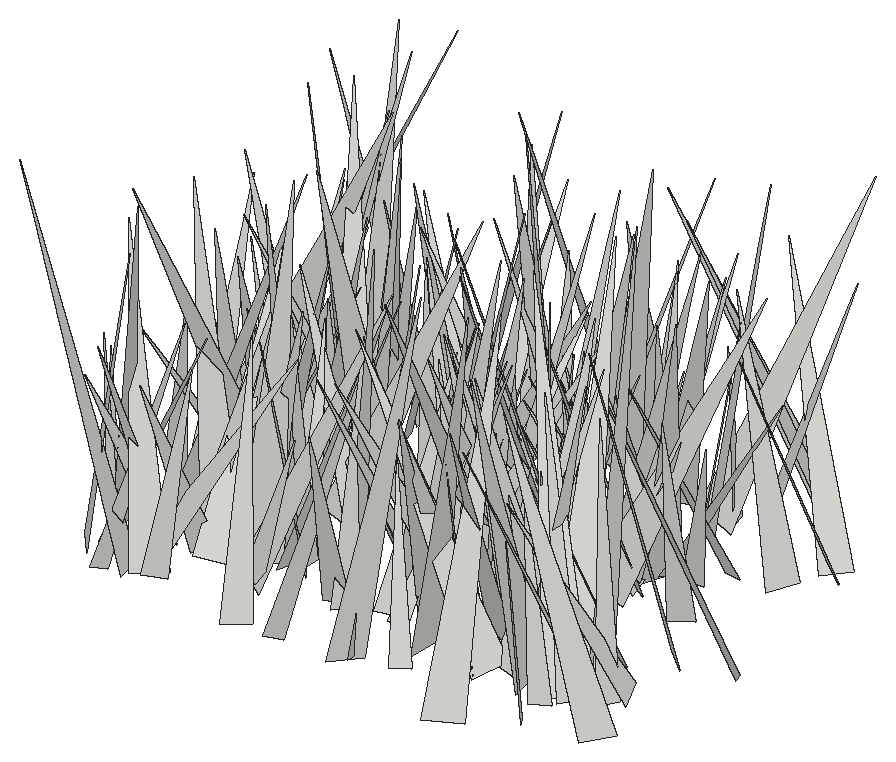
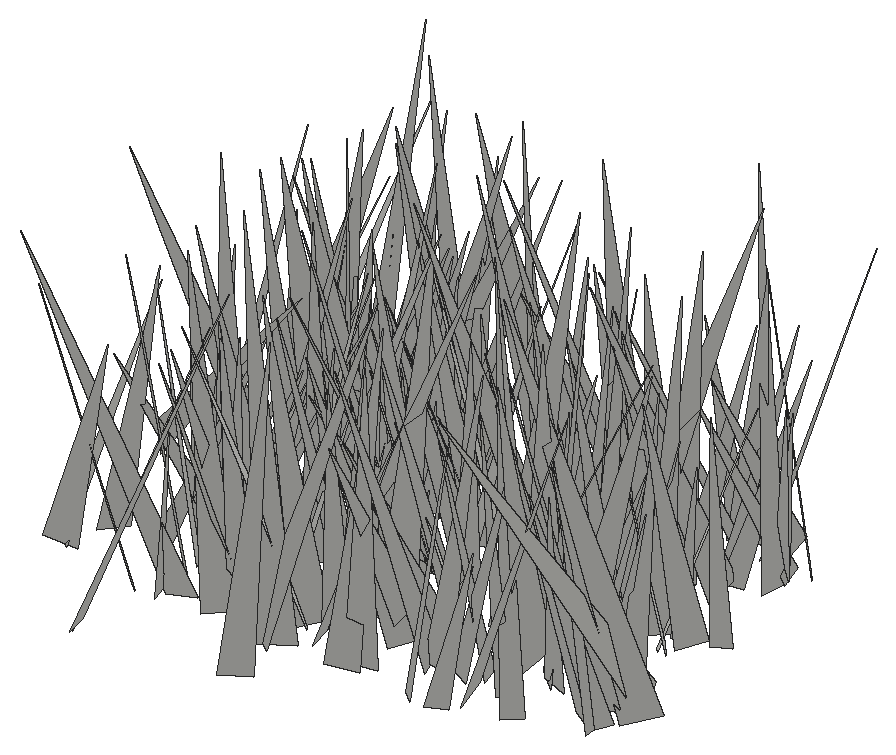
# SketchUp Ruby script. Lengths in inches.
U = 1.inch
M = Sketchup.active_model
def pt(a) = Geom::Point3d.new(a.map { |v| v * U })
def face(e, loops, mat)
  f = e.add_face(loops[0].map { |a| pt(a) })
  loops[1..].each { |l| e.add_face(l.map { |a| pt(a) }).erase! }
  f.material = f.back_material = mat if mat
  f
end
# faces: each face lists its corners as indices into pts; further lists are holes
def faces(e, pts, list, mat = nil) = list.each { |f| face(e, (f[0].is_a?(Array) ? f : [f]).map { |l| l.map { |i| pts[i] } }, mat) }
# xy, xz, yz: faces in a plane at the given z, y or x. An outline is a flat list of corners, or four numbers for a rectangle; further outlines are holes
def ring(l) = l.size == 4 ? [[l[0], l[1]], [l[2], l[1]], [l[2], l[3]], [l[0], l[3]]] : l.each_slice(2).to_a
def flat(e, list, mat, &to3) = list.each { |f| face(e, (f[0].is_a?(Array) ? f : [f]).map { |l| ring(l).map { |u, v| to3.(u, v) } }, mat) }
def xy(e, z, list, mat = nil) = flat(e, list, mat) { |x, y| [x, y, z] }
def xz(e, y, list, mat = nil) = flat(e, list, mat) { |x, z| [x, y, z] }
def yz(e, x, list, mat = nil) = flat(e, list, mat) { |y, z| [x, y, z] }
def lines(e, pts, list) = list.each { |a, b| e.add_line(pt(pts[a]), pt(pts[b])) }
# prism: a flat outline (further loops are holes) pulled along v
def prism(e, loops, v, mat = nil)
  f = face(e, loops, mat); d = Geom::Vector3d.new(v.map { |x| x * U })
  f.pushpull(f.normal.samedirection?(d) ? d.length : -d.length)
end
def box(e, o, s, mat = nil) = prism(e, [[o, [o[0] + s[0], o[1], o[2]], [o[0] + s[0], o[1] + s[1], o[2]], [o[0], o[1] + s[1], o[2]]]], [0, 0, s[2]], mat)
def at(x, y, z, deg = 0) = Geom::Transformation.translation(pt([x, y, z])) * Geom::Transformation.rotation(ORIGIN, Z_AXIS, deg.degrees)
def axes(o, x, y, z) = Geom::Transformation.new([*x, 0, *y, 0, *z, 0, *pt(o).to_a, 1])
def part(name) = M.definitions.add(name)
# library, detail: a bought-in or finely detailed component or shape, given as its bounding box
def library(name, o, s) = part(name).tap { |d| box(d.entities, o, s) }
def detail(e, o, s) = box(e.add_group.entities, o, s)
def put(e, d, t, mat = nil) = e.add_instance(d, t).tap { |i| i.material = mat if mat }
def group(e, t, mat = nil) = e.add_group.tap { |g| g.transformation = t; g.material = mat if mat }.entities
root = M.entities
c1 = part("fur_instance\#9")
p = [[0.8125,0,1.79],[0.67,-0.02,1.48],[0,-0.11,0],[0,0.11,0]]
faces(c1.entities,p,[[0,1,2,3]])
put(root,c1,axes([133.73,308.41,-27.1],[-4.47092,-4.93614,0.16266],[-4.90041,4.46105,0.68268],[0.61475,-0.33851,6.62484]))
put(root,c1,axes([114.86,306.08,-27.1],[-2.17172,3.54056,2.13295],[3.72846,2.71807,-0.7156],[1.78427,-1.37037,4.09143]))
put(root,c1,axes([130.49,308.72,-27.1],[7.53052,-1.13144,2.64431],[-0.30654,-7.68469,-2.41514],[-2.85982,-2.15562,7.22191]))
put(root,c1,axes([113.78,305.95,-27.1],[-7.70081,-2.50661,0.76749],[-2.60656,7.57519,-1.4131],[0.27927,1.58364,7.97425]))
put(root,c1,axes([119.4,305.24,-27.1],[3.60121,-2.60608,3.3834],[-3.59297,-4.24118,0.55747],[-2.30861,2.53545,4.41017]))
put(root,c1,axes([132.16,306.06,-27.1],[-3.20539,-1.99252,1.2784],[-2.28309,3.17085,-0.78241],[0.62603,1.36182,3.69222]))
put(root,c1,axes([135.17,306.77,-27.1],[-3.75455,5.21199,1.89568],[5.51913,3.28609,1.89629],[-0.5456,-2.62523,6.13723]))
put(root,c1,axes([124.23,305.61,-27.1],[6.87844,-2.02965,2.77665],[-2.6588,-7.07628,1.41394],[-2.18175,2.22463,7.03088]))
put(root,c1,axes([111.28,306.52,-27.1],[4.60486,4.04407,1.88978],[4.30358,-4.74303,-0.33665],[-1.18533,-1.50984,6.1193]))
put(root,c1,axes([113.47,308.5,-27.1],[-0.2394,-4.99537,0.47277],[-5.01072,0.21306,-0.28607],[-0.26442,0.48521,4.99291]))
put(root,c1,axes([129.92,304.25,-27.1],[-5.97227,4.9002,0.90124],[4.6479,5.98621,-1.7477],[1.79477,0.80344,7.52499]))
put(root,c1,axes([111.55,308.375,-27.1],[7.9282,0.66664,2.15118],[1.11346,-8.00329,-1.62351],[-1.9576,-1.85234,7.78877]))
put(root,c1,axes([114.93,308.92,-27.1],[3.23703,-3.40023,0.62778],[-3.13183,-3.24768,-1.44163],[-1.46538,-0.57015,4.46784]))
put(root,c1,axes([112.91,309.12,-27.1],[3.29812,-3.00828,0.87507],[-2.53709,-3.30998,-1.81667],[-1.83812,-0.82908,4.07763]))
put(root,c1,axes([121.28,308.8,-27.1],[1.53045,-4.60076,0.23907],[-4.60681,-1.52625,0.11946],[0.03806,0.26453,4.84716]))
put(root,c1,axes([114.52,306.23,-27.1],[-3.46559,5.8146,1.30946],[5.95968,3.40104,0.67057],[0.08042,-1.46897,6.73574]))
put(root,c1,axes([126.2,306.37,-27.1],[-1.47936,3.73163,0.54523],[3.76451,1.42617,0.45319],[-0.22551,-0.67216,3.98851]))
put(root,c1,axes([128.33,307.89,-27.1],[-3.06281,-3.15709,1.43812],[-3.29391,3.24851,0.11628],[1.08883,0.94666,4.3971]))
put(root,c1,axes([127.84,310.375,-27.1],[-0.91329,-6.82842,0.06821],[-6.63421,0.90353,1.6239],[1.61843,-0.14959,6.69511]))
put(root,c1,axes([112.84,305.34,-27.1],[4.59265,0.40937,1.72839],[-0.43371,-4.3881,2.19176],[-1.72245,2.19644,4.05662]))
put(root,c1,axes([125.98,308.26,-27.1],[7.89082,-0.9052,1.78608],[-0.78265,-8.07818,-0.63641],[-1.84308,-0.44515,7.91703]))
put(root,c1,axes([113.76,307.28,-27.1],[3.2036,5.15972,0.63397],[4.7617,-2.61371,-2.78969],[2.08586,-1.95793,5.39475]))
put(root,c1,axes([131.92,307.42,-27.1],[-1.38179,3.78074,1.32931],[4.00762,1.30133,0.46468],[-0.00636,-1.40818,3.99842]))
put(root,c1,axes([112.24,306.98,-27.1],[0.5553,3.90242,1.15183],[3.90207,-0.84018,0.96535],[-1.15302,-0.96393,3.8217]))
put(root,c1,axes([117.9,308.01,-27.1],[1.20072,-3.47995,0.99765],[-3.52529,-0.88496,1.15597],[0.82322,1.28603,3.49507]))
put(root,c1,axes([111.97,307.41,-27.1],[0.50374,3.60666,1.32904],[3.78488,-0.69911,0.46265],[-0.67011,-1.23747,3.61216]))
put(root,c1,axes([128.89,308.32,-27.1],[-6.43604,2.78332,0.65453],[2.85741,6.20344,1.71766],[-0.1023,-1.83529,6.79846]))
put(root,c1,axes([124.49,310.56,-27.1],[6.011,-2.52803,0.45147],[-2.2406,-5.7244,-2.22212],[-1.25478,-1.8887,6.13068]))
put(root,c1,axes([134.04,310.125,-27.1],[-4.91943,-1.92287,0.32626],[-1.70701,4.67316,1.80343],[0.9434,-1.57124,4.96446]))
put(root,c1,axes([126.09,310.48,-27.1],[4.34994,-4.04005,0.73934],[-3.73736,-4.34022,-1.72779],[-1.70317,-0.79441,5.67968]))
put(root,c1,axes([121.12,305.25,-27.1],[5.49101,0.89671,2.25711],[-0.37206,-5.20349,2.97239],[-2.40004,2.85822,4.70322]))
put(root,c1,axes([124.3,306.1,-27.1],[-6.72177,-1.11045,3.37602],[-2.29516,6.87097,-2.30972],[2.71346,3.06096,6.4094]))
put(root,c1,axes([125.15,311.5,-27.1],[-6.3203,-1.31951,1.76492],[-0.3807,5.93404,3.07318],[2.17051,-2.80147,5.67828]))
put(root,c1,axes([111.65,307.2,-27.1],[4.45385,0.90104,0.34779],[0.77968,-4.32278,1.21461],[-0.57002,1.12752,4.37874]))
put(root,c1,axes([117.67,308.17,-27.1],[3.41975,6.53108,1.33927],[6.45057,-2.86091,-2.51965],[1.68487,-2.30293,6.92828]))
put(root,c1,axes([123.74,311.39,-27.1],[-5.24067,-3.21189,0.67738],[-2.84495,5.08085,2.08111],[1.63749,-1.45206,5.78359]))
put(root,c1,axes([121.59,309.46,-27.1],[-3.32783,-6.52848,3.29816],[-6.89122,4.01297,0.99019],[2.45153,2.41834,7.26051]))
put(root,c1,axes([118.82,310.05,-27.1],[-3.91635,-3.27614,1.36892],[-3.24396,4.13005,0.60351],[1.44353,0.39293,5.07017]))
put(root,c1,axes([121.82,308.65,-27.1],[4.3952,-2.19196,2.60814],[-2.70598,-4.83259,0.49862],[-2.06997,1.6632,4.88608]))
put(root,c1,axes([123.3,310.01,-27.1],[3.09975,-1.98369,0.33098],[-1.98147,-3.11644,-0.1208],[-0.34401,0.07615,3.67817]))
put(root,c1,axes([117.23,309.3,-27.1],[-5.12716,5.45276,3.67809],[5.84452,5.9162,-0.62364],[3.01704,-2.19425,7.45865]))
put(root,c1,axes([132.65,308.37,-27.1],[-5.52094,1.92393,0.48296],[1.85996,5.5174,-0.71721],[0.68943,0.52184,5.80241]))
put(root,c1,axes([129.99,309.48,-27.1],[5.84499,-0.86217,1.83487],[-1.09003,-6.05756,0.62599],[-1.70936,0.91471,5.87498]))
put(root,c1,axes([116.05,310.88,-27.1],[3.45559,-4.90486,0.92565],[-4.98413,-3.32981,0.96246],[0.2699,1.30779,5.9222]))
put(root,c1,axes([118.2,309.93,-27.1],[6.4862,-0.82849,0.61771],[-0.87391,-6.49276,0.46816],[-0.55158,0.54452,6.52212]))
put(root,c1,axes([124.09,308.82,-27.1],[-0.30009,3.62925,0.24074],[3.53668,0.34756,-0.831],[0.84929,-0.16496,3.54556]))
put(root,c1,axes([115.39,312.97,-27.1],[0.76231,-8.24421,0.75454],[-8.09051,-0.90251,-1.68715],[-1.75496,0.57958,8.10565]))
put(root,c1,axes([133.84,309.01,-27.1],[-5.20641,1.3754,0.94823],[1.21962,5.25029,-0.91901],[1.14166,0.66356,5.30602]))
put(root,c1,axes([132.34,308.51,-27.1],[-4.81407,6.51041,0.79127],[6.55623,4.75265,0.78417],[-0.16528,-1.10168,8.05889]))
put(root,c1,axes([114.375,309.32,-27.1],[1.48764,5.46016,1.29529],[5.56167,-1.25605,-1.09283],[0.74757,-1.52092,5.55267]))
put(root,c1,axes([129.38,308.63,-27.1],[1.31333,6.20143,0.89],[6.24264,-1.21867,-0.72041],[0.52849,-1.01577,6.2979]))
put(root,c1,axes([114.73,310.27,-27.1],[-4.39266,5.33205,2.64396],[5.82364,4.52851,0.54275],[1.2274,-2.40386,6.88706]))
put(root,c1,axes([125.45,313.41,-27.1],[-0.22294,-7.81188,0.28991],[-7.80547,0.20653,-0.4373],[-0.42917,0.30182,7.80282]))
put(root,c1,axes([123.33,309.29,-27.1],[-3.03856,4.16793,1.35783],[3.96538,3.31773,-1.3102],[1.86846,-0.26309,4.98878]))
put(root,c1,axes([128.83,311.73,-27.1],[2.48728,-3.44318,0.65298],[-3.47724,-2.52444,-0.0662],[-0.43662,0.49004,4.24707]))
put(root,c1,axes([127.87,310.9,-27.1],[-1.21907,-3.82959,1.50139],[-4.09681,0.98993,-0.80143],[-0.36895,1.66143,3.93822]))
put(root,c1,axes([115.7,308.37,-27.1],[-3.21539,5.33291,0.27404],[5.21793,3.20577,-1.16191],[1.13501,0.36996,6.11789]))
put(root,c1,axes([117.01,311.65,-27.1],[-6.68895,-1.28776,2.75903],[-1.15,7.23488,0.5888],[2.81923,-0.10417,6.78629]))
put(root,c1,axes([118.74,310.32,-27.1],[-5.92753,-0.80933,1.51712],[-1.07571,5.99367,-1.00549],[1.34146,1.2301,5.89742]))
put(root,c1,axes([129.59,310.8,-27.1],[4.46233,4.90899,2.88894],[5.22756,-4.98695,0.39938],[-2.26203,-1.84084,6.62202]))
put(root,c1,axes([132.49,311.65,-27.1],[-2.45002,-3.17903,0.27674],[-3.09062,2.27713,-1.20338],[-0.79426,0.94543,3.82893]))
put(root,c1,axes([114.55,311.58,-27.1],[3.71133,-3.4553,1.19556],[-3.62183,-3.7076,0.52772],[-0.50083,1.20708,5.04327]))
put(root,c1,axes([124.94,311.71,-27.1],[2.55776,-3.86723,2.22173],[-4.13899,-3.01226,-0.47827],[-1.66143,1.55064,4.61182]))
put(root,c1,axes([129.2,310.5,-27.1],[-3.21117,5.73542,2.2751],[5.803,3.67883,-1.08356],[2.09673,-1.39782,6.48325]))
put(root,c1,axes([128.78,311.85,-27.1],[-0.87207,-5.64239,2.10409],[-5.67136,0.05471,-2.20385],[-2.02471,2.277,5.26688]))
put(root,c1,axes([127.8,312.64,-27.1],[-5.01187,1.13995,1.85475],[1.60842,5.07616,1.22637],[1.46717,-1.67079,4.99142]))
put(root,c1,axes([121.78,311.68,-27.1],[5.2265,3.38981,1.10604],[3.55749,-5.09026,-1.20993],[-0.2416,-1.62138,6.11091]))
put(root,c1,axes([123.86,311.71,-27.1],[1.63751,6.97927,2.94123],[7.53115,-1.18196,-1.38823],[0.80173,-3.15202,7.03309]))
put(root,c1,axes([126.96,310.5,-27.1],[1.83922,3.08635,0.93557],[2.6886,-2.06216,1.51739],[-1.78108,0.07419,3.25666]))
put(root,c1,axes([133.74,313.15,-27.1],[-4.39451,-5.32367,1.29551],[-5.40377,4.48556,0.10243],[0.905,0.93264,6.90237]))
put(root,c1,axes([112.91,309.66,-27.1],[7.28027,0.47928,1.68125],[-0.05604,-7.13268,2.27604],[-1.74733,2.22571,6.93193]))
put(root,c1,axes([126.48,312.2,-27.1],[0.21554,-5.31829,2.18174],[-5.56977,-0.73327,-1.23719],[-1.42193,2.0661,5.17688]))
put(root,c1,axes([112.05,314.6,-27.1],[-3.67716,-3.23058,0.06887],[-2.92053,3.36739,2.02339],[1.38271,-1.47883,4.45691]))
put(root,c1,axes([125.39,314.32,-27.1],[2.94915,-5.28887,0.70098],[-5.06545,-3.02722,-1.5291],[-1.67475,-0.15728,5.85931]))
put(root,c1,axes([110.33,312.99,-27.1],[0.87128,-4.23502,0.75689],[-4.24446,-0.72019,0.85631],[0.702,0.90186,4.23807]))
put(root,c1,axes([120.27,313.47,-27.1],[-1.91573,-3.10975,0.18965],[-3.07242,1.92263,0.49017],[0.51647,-0.09744,3.61944]))
put(root,c1,axes([112.78,313.71,-27.1],[5.63565,-3.00774,1.4531],[-2.80235,-5.80815,-1.15361],[-1.81792,-0.37081,6.28301]))
put(root,c1,axes([114.55,312.53,-27.1],[-3.7389,-0.44853,0.79303],[-0.43438,3.82202,0.11371],[0.80087,-0.02096,3.764]))
put(root,c1,axes([122.02,312.58,-27.1],[0.68635,-5.64905,2.27441],[-5.90756,-0.06201,1.6287],[1.47832,2.3749,5.45254]))
put(root,c1,axes([123.22,311.27,-27.1],[3.32598,3.77438,0.4675],[3.78797,-3.34308,0.04133],[-0.34022,-0.32329,5.03054]))
put(root,c1,axes([117.91,311.31,-27.1],[-3.18277,2.93848,0.48438],[2.88307,3.21784,-0.5768],[0.74643,0.10079,4.29324]))
put(root,c1,axes([131.42,309.86,-27.1],[-6.0602,5.67803,0.65626],[5.53411,6.06799,-1.39639],[1.4298,0.57987,8.18634]))
put(root,c1,axes([122.61,312.87,-27.1],[4.92372,-1.23429,0.65682],[-1.32256,-4.89156,0.72207],[-0.45359,0.86432,5.02445]))
put(root,c1,axes([111.84,313.5,-27.1],[0.6335,-3.36408,1.34348],[-3.58683,-0.77327,-0.24494],[-0.50657,1.2682,3.41444]))
put(root,c1,axes([128.84,315.43,-27.1],[-3.83157,-3.11067,0.41222],[-2.87249,3.73899,1.51524],[1.26294,-0.9332,4.69694]))
put(root,c1,axes([120.3,316.05,-27.1],[-2.61623,-5.06997,0.16776],[-4.93297,2.58676,1.24576],[1.18261,-0.42604,5.56752]))
put(root,c1,axes([118.55,313.63,-27.1],[-3.73959,3.61146,1.09906],[3.77498,3.58144,1.07604],[0.00944,-1.53809,5.08619]))
put(root,c1,axes([131.83,311.15,-27.1],[-7.99125,0.08509,2.25297],[-0.74491,7.73167,-2.93422],[2.12796,3.02611,7.43355]))
put(root,c1,axes([117.53,313.63,-27.1],[1.82991,-7.19945,3.13467],[-7.38413,-0.48301,3.20126],[2.67073,3.59742,6.70317]))
put(root,c1,axes([129.05,316.58,-27.1],[-2.89154,-5.8907,0.51675],[-5.81601,2.937,0.93617],[1.06836,0.04534,6.49499]))
put(root,c1,axes([136.35,313.55,-27.1],[-4.35257,-4.39527,0.35538],[-3.69396,3.36161,-3.66659],[-2.40819,2.78761,4.98191]))
put(root,c1,axes([124.13,317.67,-27.1],[-3.49524,-7.20934,0.56433],[-6.86604,3.50524,2.25399],[2.26947,-0.49846,7.68835]))
put(root,c1,axes([113.61,315,-27.1],[5.71322,-0.96407,0.62556],[-0.92485,-5.73993,-0.39936],[-0.68221,-0.29224,5.7802]))
put(root,c1,axes([117.31,316.57,-27.1],[6.25935,-4.83068,2.00086],[-4.50057,-6.56633,-1.77386],[-2.66155,-0.25726,7.70509]))
put(root,c1,axes([127.67,314.96,-27.1],[-4.9951,-5.23204,0.99068],[-5.30492,4.77148,-1.54841],[-0.46216,1.77916,7.06595]))
put(root,c1,axes([132.0625,315.59,-27.1],[2.34766,-4.1804,1.05082],[-4.25289,-2.44131,-0.21062],[-0.70205,0.80976,4.78987]))
put(root,c1,axes([126.87,316.02,-27.1],[1.30695,-5.86281,0.96642],[-5.89292,-1.15208,0.98022],[0.76158,1.14664,5.9262]))
put(root,c1,axes([111.87,314.36,-27.1],[3.13745,2.7412,0.96065],[2.81213,-3.22064,0.00574],[-0.7273,-0.62763,4.16626]))
put(root,c1,axes([111.26,313.54,-27.1],[-4.2045,3.84796,1.64776],[3.68267,4.51063,-1.13666],[1.98995,-0.21727,5.58504]))
put(root,c1,axes([129.21,316.73,-27.1],[-4.78281,-0.5343,0.54387],[-0.29464,4.48183,1.81189],[0.70318,-1.75621,4.45846]))
put(root,c1,axes([114.99,315.49,-27.1],[6.44965,-0.53992,1.19924],[-0.48241,-6.55498,-0.35669],[-1.22351,-0.26161,6.46237]))
put(root,c1,axes([122.49,315.66,-27.1],[4.00541,-4.88826,1.49079],[-5.10449,-3.91872,0.86522],[-0.24835,1.7057,6.26017]))
put(root,c1,axes([113.32,316.55,-27.1],[-1.78915,-3.44674,0.35763],[-3.41457,1.82215,0.479],[0.59044,0.09337,3.85378]))
put(root,c1,axes([111.07,317.39,-27.1],[4.81338,-2.70132,0.36004],[-2.51999,-4.69011,-1.49931],[-1.0375,-1.14068,5.31205]))
put(root,c1,axes([117.125,317.07,-27.1],[-5.82237,-2.50943,0.01956],[-2.48564,5.77362,0.82736],[0.34528,-0.75212,6.28591]))
put(root,c1,axes([122.29,314.95,-27.1],[3.35941,2.47012,0.56366],[2.52325,-3.34641,-0.37364],[-0.22894,-0.63632,4.15301]))
put(root,c1,axes([115.23,316.26,-27.1],[1.42662,-4.11071,0.89066],[-4.20545,-1.41051,0.22612],[-0.07357,0.91596,4.34535]))
put(root,c1,axes([120.125,315.75,-27.1],[-0.91503,4.79321,2.31879],[5.31141,0.98733,0.05504],[0.37492,-2.28894,4.87946]))
put(root,c1,axes([121.08,318.71,-27.1],[6.38764,-4.10189,0.26345],[-3.90919,-6.21298,-1.95294],[-1.27011,-1.50671,7.33577]))
put(root,c1,axes([113.18,314.32,-27.1],[4.04294,1.47662,0.10602],[1.40514,-3.92456,1.07725],[-0.46609,0.97696,4.16717]))
put(root,c1,axes([122.45,315.18,-27.1],[3.25743,4.86298,0.41292],[4.6269,-2.91916,-2.12138],[1.55271,-1.50328,5.4552]))
put(root,c1,axes([122.65,317.02,-27.1],[1.67883,-4.20753,0.33675],[-4.18563,-1.61266,0.71764],[0.54516,0.57551,4.47289]))
put(root,c1,axes([124.76,316.9375,-27.1],[-6.87538,0.87455,0.95023],[1.06547,6.75006,1.49673],[0.72976,-1.61573,6.76724]))
put(root,c1,axes([115.11,315.92,-27.1],[4.62251,0.92588,0.22465],[0.9419,-4.60847,-0.38752],[-0.14333,-0.42437,4.69837]))
put(root,c1,axes([114.61,315.9,-27.1],[0.94645,-5.69848,3.07489],[-6.04954,-1.88624,-1.63358],[-2.30884,2.60631,5.54074]))
put(root,c1,axes([129.4375,317.72,-27.1],[6.44633,-3.37101,0.63256],[-3.2949,-6.46051,-0.8512],[-0.95262,-0.46602,7.22457]))
put(root,c1,axes([117.5,315.53,-27.1],[3.62939,6.32437,2.66269],[6.74766,-3.83695,-0.08396],[-1.24771,-2.35377,7.2913]))
put(root,c1,axes([125.81,319.31,-27.1],[-3.26721,-5.06008,0.08616],[-4.54982,2.98181,2.58736],[2.21606,-1.33826,5.43917]))
put(root,c1,axes([128.86,316.43,-27.1],[3.23817,-2.36152,0.30304],[-2.37388,-3.16317,0.7165],[0.18248,0.75624,3.94324]))
put(root,c1,axes([126.04,317.25,-27.1],[3.30583,-2.31707,0.74955],[-2.21165,-3.38553,-0.71128],[-1.01942,-0.16893,3.97384]))
put(root,c1,axes([128.5,315.48,-27.1],[2.77972,-6.83526,2.99642],[-7.05556,-1.36449,3.4327],[2.43278,3.85274,6.53179]))
put(root,c1,axes([123.89,314.84,-27.1],[3.6487,6.36792,1.23917],[6.47764,-3.65398,-0.29593],[-0.35515,-1.22351,7.3332]))
put(root,c1,axes([125.69,315.8125,-27.1],[2.40724,3.27999,1.19788],[3.2967,-2.61439,0.53362],[-1.15108,-0.62824,4.03341]))
put(root,c1,axes([113.14,315.72,-27.1],[-4.26519,0.30143,0.24037],[0.24291,4.17451,-0.92459],[0.29939,0.9072,4.17466]))
put(root,c1,axes([119.33,317.12,-27.1],[3.22787,2.03353,0.24614],[1.96333,-2.94045,-1.45397],[0.58408,-1.35405,3.52709]))
put(root,c1,axes([124.96,316.69,-27.1],[2.68991,-2.47286,1.2383],[-2.72716,-2.65872,0.6147],[-0.45937,1.30393,3.60178]))
put(root,c1,axes([130.63,318.06,-27.1],[1.50872,-3.69838,0.31644],[-3.67115,-1.43625,0.71715],[0.54852,0.55997,3.92937]))
put(root,c1,axes([122.6,315.3,-27.1],[-0.90144,4.87523,0.09791],[4.65666,0.89022,-1.45364],[1.44671,0.1723,4.73998]))
put(root,c1,axes([120.81,315.94,-27.1],[5.6278,2.51424,1.57514],[2.22036,-5.80941,1.3399],[-1.96786,0.63554,6.01649]))
put(root,c1,axes([127.95,317.5625,-27.1],[-0.77592,-4.15559,2.31409],[-4.39268,1.52537,1.26634],[1.82437,1.90534,4.03328]))
put(root,c1,axes([113.79,318.87,-27.1],[-5.15951,-5.90719,2.53837],[-5.9684,5.61072,0.92562],[2.3909,1.25844,7.78837]))
put(root,c1,axes([129.41,317.875,-27.1],[-1.9475,3.70978,1.3462],[3.85912,1.47603,1.51527],[-0.82582,-1.85103,3.9063]))
put(root,c1,axes([131.45,319.39,-27.1],[-1.6318,-4.41068,0.10105],[-4.3461,1.58854,-0.8456],[-0.75876,0.38671,4.62621]))
put(root,c1,axes([115.875,316.5,-27.1],[-4.53452,6.13099,1.20513],[6.2123,4.58336,0.05748],[0.66981,-1.00349,7.62546]))
put(root,c1,axes([119.76,317.56,-27.1],[-4.39525,1.44739,0.73649],[1.42922,4.45652,-0.22883],[0.77116,-0.01,4.62177]))
put(root,c1,axes([126.78,318.08,-27.1],[0.00954,3.59248,1.3323],[3.47361,-0.5704,1.51319],[-1.6171,-1.20405,3.25826]))
put(root,c1,axes([128.93,319.07,-27.1],[-2.91318,-3.12111,0.33199],[-3.12229,2.8354,-0.74159],[-0.32068,0.74655,4.20452]))
put(root,c1,axes([127.3,318.16,-27.1],[6.46627,-2.11143,1.67342],[-2.36842,-6.52888,0.91405],[-1.28416,1.40953,6.74057]))
put(root,c1,axes([109.21,319.0625,-27.1],[3.50419,-7.42751,1.71848],[-7.22357,-2.63012,3.36199],[2.43745,2.88357,7.49295]))
put(root,c1,axes([129.51,317.94,-27.1],[4.38555,-0.36882,0.03632],[-0.36139,-4.16033,1.38975],[0.08213,1.3878,4.17584]))
put(root,c1,axes([112.98,321.96,-27.1],[-1.84089,-7.99139,1.4242],[-7.16502,2.28604,3.56596],[3.81486,0.4373,7.3848]))
put(root,c1,axes([112.15,318.21,-27.1],[3.861,5.57007,1.34937],[5.71182,-3.87341,-0.35436],[-0.47072,-1.31331,6.76812]))
put(root,c1,axes([119.64,320.15,-27.1],[2.07826,-5.21506,0.82935],[-4.82149,-1.51054,2.58366],[2.15357,1.65083,4.98405]))
put(root,c1,axes([124.36,321.22,-27.1],[-2.66612,-3.28273,0.28859],[-3.19335,2.6653,0.81637],[0.81369,-0.29607,4.14946]))
put(root,c1,axes([124.3,317.71,-27.1],[2.11808,6.39246,0.96016],[6.39192,-2.22182,0.69185],[-0.96378,-0.68681,6.6986]))
put(root,c1,axes([129.39,319.92,-27.1],[4.62058,2.87983,1.50344],[3.15499,-4.60106,-0.88304],[-0.77446,-1.56215,5.37246]))
put(root,c1,axes([117.57,320.7,-27.1],[-0.73911,-5.79285,1.55471],[-5.99778,0.70592,-0.22109],[-0.03032,1.57006,5.83563]))
put(root,c1,axes([123.41,318.99,-27.1],[-6.49961,-2.89491,2.26898],[-3.37847,6.5202,-1.35892],[1.4542,2.20912,6.98418]))
put(root,c1,axes([110.62,319.27,-27.1],[0.08637,4.97569,1.67082],[5.15736,0.22998,-0.95146],[0.97504,-1.65717,4.88463]))
put(root,c1,axes([128.4,318.73,-27.1],[-0.17119,5.69768,1.30234],[5.83131,0.07859,0.42267],[-0.39436,-1.31119,5.68456]))
put(root,c1,axes([133.4,319.87,-27.1],[-5.24229,2.67543,1.59997],[2.88849,5.34612,0.52444],[1.17239,-1.20849,5.86212]))
put(root,c1,axes([134.33,321.72,-27.1],[-3.22391,-4.50813,0.36238],[-4.51102,3.23719,0.13952],[0.32445,0.21334,5.54053]))
put(root,c1,axes([113.35,319.03,-27.1],[0.59003,4.76484,1.13067],[4.77949,-0.80843,0.91275],[-1.06703,-0.9864,4.71367]))
put(root,c1,axes([115.65,319.95,-27.1],[4.51759,1.55237,1.02195],[1.60919,-4.61101,-0.10928],[-0.92991,-0.4377,4.77562]))
put(root,c1,axes([114.1,320.96,-27.1],[-0.90647,-5.11686,1.80724],[-5.12934,1.40604,1.40817],[1.7715,1.45288,5.00209]))
put(root,c1,axes([110.01,320.47,-27.1],[2.80159,-3.67069,0.58517],[-3.61323,-2.51742,1.50747],[0.87232,1.36159,4.36468]))
put(root,c1,axes([110.16,320.83,-27.1],[5.07227,1.20948,1.05659],[1.39553,-5.05165,-0.91676],[-0.7948,-1.15114,5.13326]))
put(root,c1,axes([126.54,321.58,-27.1],[1.54796,-4.76639,0.70367],[-4.81569,-1.50748,0.38266],[0.1508,0.78667,4.99682]))
put(root,c1,axes([116.57,320.64,-27.1],[-1.858,-4.3991,1.45242],[-4.62148,1.65138,-0.9103],[-0.32175,1.68364,4.68782]))
put(root,c1,axes([119.65,317.87,-27.1],[4.83042,2.64277,1.00625],[2.0268,-4.62442,2.4159],[-1.97202,1.72053,4.9478]))
put(root,c1,axes([123.18,320.98,-27.1],[5.25974,-3.61511,1.15521],[-3.73911,-5.27428,0.51907],[-0.65007,1.0869,6.36116]))
put(root,c1,axes([126.36,322.37,-27.1],[4.17782,-5.39394,0.17375],[-5.37681,-4.14138,0.71959],[0.46328,0.57738,6.78461]))
put(root,c1,axes([122.23,320.7,-27.1],[-2.98009,3.50221,2.17702],[3.82104,3.35523,-0.16707],[1.55067,-1.53712,4.59549]))
put(root,c1,axes([114.94,318.15,-27.1],[-7.79963,1.89477,1.60693],[1.33324,7.65978,-2.56065],[2.09639,2.17814,7.60707]))
put(root,c1,axes([127.8,319.33,-27.1],[5.12063,-0.00436,1.95562],[-0.62511,-5.19742,1.62522],[-1.85303,1.74129,4.85588]))
put(root,c1,axes([110.86,320.4375,-27.1],[4.61104,6.12434,1.67223],[6.3457,-4.50796,-0.9879],[-0.18966,-1.93296,7.60219]))
put(root,c1,axes([125.81,321.71,-27.1],[2.0151,-5.02328,1.60572],[-5.27188,-1.87389,0.75376],[0.13771,1.76848,5.35965]))
put(root,c1,axes([122.28,321.64,-27.1],[-5.21279,-1.15752,0.50027],[-1.17064,5.23306,-0.0898],[0.46875,0.19648,5.33901]))
put(root,c1,axes([120.24,322.9,-27.1],[1.37866,-6.43403,1.32521],[-6.55871,-1.42426,-0.09169],[-0.36909,1.27608,6.57944]))
put(root,c1,axes([123.24,322.99,-27.1],[1.49707,-8.01218,1.60299],[-8.01526,-1.12338,1.87068],[1.58751,1.88383,7.93327]))
put(root,c1,axes([109.92,317.76,-27.1],[7.75154,3.11882,0.30174],[2.75499,-7.16733,3.30818],[-1.4927,2.96765,7.67264]))
put(root,c1,axes([115.31,321.52,-27.1],[-7.20158,-1.52489,0.67202],[-1.60184,7.15641,-0.92717],[0.45935,1.04894,7.30263]))
put(root,c1,axes([117.04,323.03,-27.1],[-3.29784,-3.61715,1.25797],[-3.53735,3.51322,0.8285],[1.46745,0.33986,4.82422]))
put(root,c1,axes([119.68,319.25,-27.1],[-3.94963,4.34285,0.40783],[4.0226,3.83915,-1.92507],[1.68683,1.01332,5.54563]))
put(root,c1,axes([124.15,322.9,-27.1],[-4.11377,-6.51171,1.45116],[-6.65439,3.88319,-1.43913],[-0.47668,1.98739,7.56666]))
put(root,c1,axes([118.02,320.34,-27.1],[6.46332,2.41268,1.62775],[2.03661,-6.58136,1.66821],[-2.07914,1.05343,6.69422]))
put(root,c1,axes([128.95,321.16,-27.1],[4.76999,5.26227,1.90717],[5.37132,-5.00824,0.38463],[-1.57405,-1.14351,7.09199]))
put(root,c1,axes([126.68,320.87,-27.1],[2.68207,4.86571,0.6841],[4.89534,-2.71316,0.10499],[-0.42283,-0.54794,5.55496]))
put(root,c1,axes([119.82,322.34,-27.1],[-1.05184,5.80364,2.59591],[6.34975,1.09094,0.13387],[0.3189,-2.57972,5.89666]))
put(root,c1,axes([123.64,320.73,-27.1],[5.3948,4.35682,0.5893],[4.31887,-5.42625,0.57994],[-0.82254,0.08385,6.9101]))
put(root,c1,axes([128.99,322.72,-27.1],[3.01328,1.01562,1.71575],[1.06477,-3.44849,0.1713],[-1.68569,-0.36275,3.17522]))
put(root,c1,axes([130.14,322.84,-27.1],[4.42305,4.26534,0.99754],[4.37397,-4.22348,-1.33498],[0.23791,-1.64944,5.99786]))
put(root,c1,axes([134.27,321.95,-27.1],[-2.5947,5.83184,0.30944],[5.66182,2.42897,1.69778],[-1.43174,-0.96349,6.15308]))
put(root,c1,axes([115.67,323.09,-27.1],[-2.80157,3.07223,0.58027],[3.12461,2.72376,0.66487],[-0.11008,-0.87559,4.10431]))
put(root,c1,axes([122.97,325.79,-27.1],[4.57924,-4.33247,0.58798],[-4.22206,-4.60304,-1.03525],[-1.13589,-0.35667,6.21836]))
put(root,c1,axes([128.25,322.3,-27.1],[1.6055,7.88479,1.47704],[7.72527,-1.11383,-2.45126],[2.16141,-1.87581,7.66412]))
put(root,c1,axes([129.89,326.47,-27.1],[-6.83596,-2.73328,0.53057],[-2.58478,6.75268,1.48423],[1.035,-1.18879,7.21098]))
put(root,c1,axes([129.98,326.38,-27.1],[-5.72076,-3.26575,0.35826],[-3.1922,5.6955,0.94426],[0.77675,-0.64548,6.51924]))
